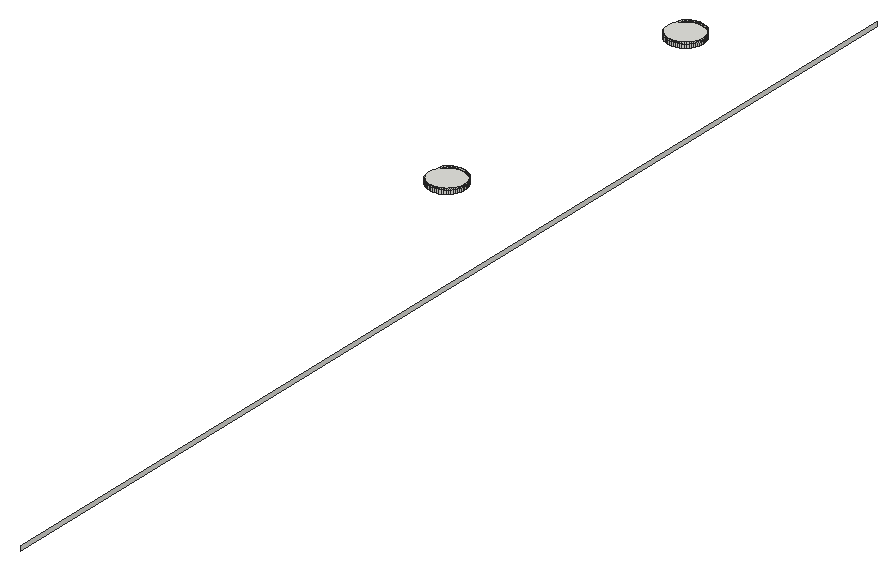
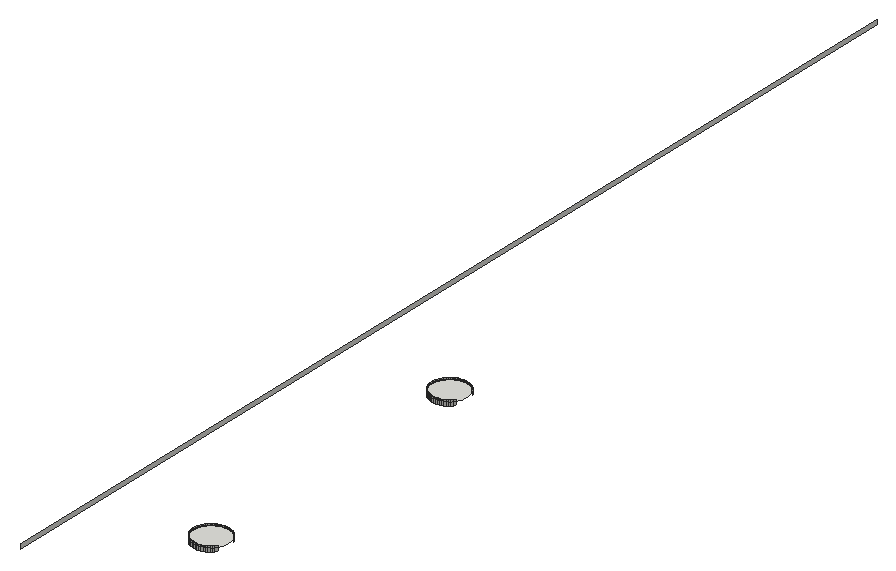
# SketchUp Ruby script. Lengths in inches.
U = 1.inch
M = Sketchup.active_model
def pt(a) = Geom::Point3d.new(a.map { |v| v * U })
def face(e, loops, mat)
  f = e.add_face(loops[0].map { |a| pt(a) })
  loops[1..].each { |l| e.add_face(l.map { |a| pt(a) }).erase! }
  f.material = f.back_material = mat if mat
  f
end
# faces: each face lists its corners as indices into pts; further lists are holes
def faces(e, pts, list, mat = nil) = list.each { |f| face(e, (f[0].is_a?(Array) ? f : [f]).map { |l| l.map { |i| pts[i] } }, mat) }
# xy, xz, yz: faces in a plane at the given z, y or x. An outline is a flat list of corners, or four numbers for a rectangle; further outlines are holes
def ring(l) = l.size == 4 ? [[l[0], l[1]], [l[2], l[1]], [l[2], l[3]], [l[0], l[3]]] : l.each_slice(2).to_a
def flat(e, list, mat, &to3) = list.each { |f| face(e, (f[0].is_a?(Array) ? f : [f]).map { |l| ring(l).map { |u, v| to3.(u, v) } }, mat) }
def xy(e, z, list, mat = nil) = flat(e, list, mat) { |x, y| [x, y, z] }
def xz(e, y, list, mat = nil) = flat(e, list, mat) { |x, z| [x, y, z] }
def yz(e, x, list, mat = nil) = flat(e, list, mat) { |y, z| [x, y, z] }
def lines(e, pts, list) = list.each { |a, b| e.add_line(pt(pts[a]), pt(pts[b])) }
# prism: a flat outline (further loops are holes) pulled along v
def prism(e, loops, v, mat = nil)
  f = face(e, loops, mat); d = Geom::Vector3d.new(v.map { |x| x * U })
  f.pushpull(f.normal.samedirection?(d) ? d.length : -d.length)
end
def box(e, o, s, mat = nil) = prism(e, [[o, [o[0] + s[0], o[1], o[2]], [o[0] + s[0], o[1] + s[1], o[2]], [o[0], o[1] + s[1], o[2]]]], [0, 0, s[2]], mat)
def at(x, y, z, deg = 0) = Geom::Transformation.translation(pt([x, y, z])) * Geom::Transformation.rotation(ORIGIN, Z_AXIS, deg.degrees)
def axes(o, x, y, z) = Geom::Transformation.new([*x, 0, *y, 0, *z, 0, *pt(o).to_a, 1])
def part(name) = M.definitions.add(name)
# library, detail: a bought-in or finely detailed component or shape, given as its bounding box
def library(name, o, s) = part(name).tap { |d| box(d.entities, o, s) }
def detail(e, o, s) = box(e.add_group.entities, o, s)
def put(e, d, t, mat = nil) = e.add_instance(d, t).tap { |i| i.material = mat if mat }
def group(e, t, mat = nil) = e.add_group.tap { |g| g.transformation = t; g.material = mat if mat }.entities
root = M.entities
xy(root,114.32,[[112.02,72.83,111.82,72.84,111.61,72.87,111.41,72.92,111.21,72.99,111.02,73.08,110.84,73.2,110.68,73.33,110.53,73.47,110.4,73.63,110.28,73.81,110.18,73.99,110.11,74.1875,110.05,74.39,110.01,74.59,110,74.8,110.01,75.01,110.04,75.22,110.09,75.42,110.16,75.62,110.26,75.81,110.37,75.98,110.5,76.15,110.64,76.3,110.8,76.43,110.98,76.55,111.16,76.65,111.36,76.72,111.56,76.78,111.77,76.8125,111.98,76.83,112.18,76.82,112.39,76.79,112.59,76.74,112.79,76.67,112.98,76.57,113.16,76.46,113.32,76.33,113.47,76.18,113.6,76.02,113.72,75.85,113.82,75.66,113.89,75.47,113.95,75.27,113.99,75.0625,114,74.85,113.99,74.64,113.96,74.4375,113.91,74.23,113.84,74.04,113.74,73.85,113.63,73.67,113.5,73.51,113.36,73.36,113.2,73.22,113.02,73.11,112.84,73.01,112.64,72.93,112.44,72.88,112.23,72.84],[112.02,106.24,111.82,106.25,111.61,106.28,111.41,106.33,111.21,106.41,111.02,106.5,110.84,106.61,110.68,106.74,110.53,106.89,110.4,107.05,110.28,107.22,110.18,107.41,110.11,107.6,110.05,107.8,110.01,108.01,110,108.22,110.01,108.43,110.04,108.63,110.09,108.84,110.16,109.03,110.26,109.22,110.37,109.4,110.5,109.5625,110.64,109.71,110.8,109.85,110.98,109.96,111.16,110.06,111.36,110.14,111.56,110.19,111.77,110.23,111.98,110.24,112.18,110.23,112.39,110.2,112.59,110.15,112.79,110.08,112.98,109.99,113.16,109.875,113.32,109.74,113.47,109.6,113.6,109.4375,113.72,109.26,113.82,109.08,113.89,108.88,113.95,108.68,113.99,108.48,114,108.27,113.99,108.06,113.96,107.85,113.91,107.65,113.84,107.45,113.74,107.26,113.63,107.09,113.5,106.92,113.36,106.77,113.2,106.64,113.02,106.52,112.84,106.43,112.64,106.35,112.44,106.29,112.23,106.26]])
yz(root,124,[[0,114,120,114.47]])
p = [[111.82,72.84,113.9],[111.61,72.87,113.9],[111.61,72.87,114.32],[111.82,72.84,114.32],[112.02,72.83,113.9],[112.02,72.83,114.32],
  [112.23,72.84,113.9],[112.23,72.84,114.32],[112.44,72.88,113.9],[112.44,72.88,114.32],[111.41,72.92,113.9],[111.21,72.99,113.9],
  [111.21,72.99,114.32],[111.41,72.92,114.32],[112.64,72.93,113.9],[112.64,72.93,114.32],[112.84,73.01,113.9],[112.84,73.01,114.32],
  [111.02,73.08,113.9],[111.02,73.08,114.32],[113.02,73.11,113.9],[113.02,73.11,114.32],[110.84,73.2,113.9],[110.84,73.2,114.32],
  [113.2,73.22,113.9],[113.2,73.22,114.32],[110.68,73.33,113.9],[110.68,73.33,114.32],[113.36,73.36,113.9],[113.36,73.36,114.32],
  [110.53,73.47,113.9],[110.53,73.47,114.32],[113.5,73.51,113.9],[113.5,73.51,114.32],[110.4,73.63,113.9],[110.4,73.63,114.32],
  [113.63,73.67,113.9],[113.63,73.67,114.32],[113.74,73.85,113.9],[113.74,73.85,114.32],[113.84,74.04,113.9],[113.84,74.04,114.32],
  [113.91,74.23,113.9],[113.91,74.23,114.32],[113.96,74.4375,113.9],[113.96,74.4375,114.32],[113.99,74.64,113.9],[113.99,74.64,114.32],
  [114,74.85,113.9],[114,74.85,114.32],[113.99,75.0625,113.9],[113.99,75.0625,114.32],[113.95,75.27,113.9],[113.95,75.27,114.32],
  [113.89,75.47,113.9],[113.89,75.47,114.32],[113.82,75.66,113.9],[113.82,75.66,114.32],[113.72,75.85,113.9],[113.72,75.85,114.32],
  [113.6,76.02,113.9],[113.6,76.02,114.32],[110.37,75.98,113.9],[110.5,76.15,113.9],[110.5,76.15,114.32],[110.37,75.98,114.32],
  [113.47,76.18,113.9],[113.47,76.18,114.32],[110.64,76.3,113.9],[110.64,76.3,114.32],[113.32,76.33,113.9],[113.32,76.33,114.32],
  [110.8,76.43,113.9],[110.8,76.43,114.32],[113.16,76.46,113.9],[113.16,76.46,114.32],[110.98,76.55,113.9],[110.98,76.55,114.32],
  [111.16,76.65,113.9],[111.16,76.65,114.32],[112.98,76.57,113.9],[112.98,76.57,114.32],[111.36,76.72,113.9],[111.36,76.72,114.32],
  [112.79,76.67,113.9],[112.79,76.67,114.32],[111.56,76.78,113.9],[111.56,76.78,114.32],[112.39,76.79,113.9],[112.59,76.74,113.9],
  [112.59,76.74,114.32],[112.39,76.79,114.32],[111.77,76.8125,113.9],[111.77,76.8125,114.32],[111.98,76.83,113.9],[111.98,76.83,114.32],
  [112.18,76.82,113.9],[112.18,76.82,114.32],[112.02,106.24,113.9],[111.82,106.25,113.9],[111.82,106.25,114.32],[112.02,106.24,114.32],
  [112.23,106.26,113.9],[112.23,106.26,114.32],[111.41,106.33,113.9],[111.21,106.41,113.9],[111.21,106.41,114.32],[111.41,106.33,114.32],
  [111.61,106.28,113.9],[111.61,106.28,114.32],[112.44,106.29,113.9],[112.44,106.29,114.32],[112.64,106.35,113.9],[112.64,106.35,114.32],
  [112.84,106.43,113.9],[112.84,106.43,114.32],[111.02,106.5,113.9],[111.02,106.5,114.32],[113.02,106.52,113.9],[113.02,106.52,114.32],
  [110.84,106.61,113.9],[110.84,106.61,114.32],[113.2,106.64,113.9],[113.2,106.64,114.32],[110.68,106.74,113.9],[110.68,106.74,114.32],
  [113.36,106.77,113.9],[113.36,106.77,114.32],[110.53,106.89,113.9],[110.53,106.89,114.32],[113.5,106.92,113.9],[113.5,106.92,114.32],
  [110.4,107.05,113.9],[110.4,107.05,114.32],[113.63,107.09,113.9],[113.63,107.09,114.32],[110.28,107.22,113.9],[110.28,107.22,114.32],
  [113.74,107.26,113.9],[113.74,107.26,114.32],[113.84,107.45,113.9],[113.84,107.45,114.32],[113.91,107.65,113.9],[113.91,107.65,114.32],
  [113.96,107.85,113.9],[113.96,107.85,114.32],[113.99,108.06,113.9],[113.99,108.06,114.32],[114,108.27,113.9],[114,108.27,114.32],
  [113.99,108.48,113.9],[113.99,108.48,114.32],[113.95,108.68,113.9],[113.95,108.68,114.32],[113.89,108.88,113.9],[113.89,108.88,114.32],
  [113.82,109.08,113.9],[113.82,109.08,114.32],[113.72,109.26,113.9],[113.72,109.26,114.32],[113.6,109.4375,113.9],[113.6,109.4375,114.32],
  [110.37,109.4,113.9],[110.5,109.5625,113.9],[110.5,109.5625,114.32],[110.37,109.4,114.32],[113.47,109.6,113.9],[113.47,109.6,114.32],
  [110.64,109.71,113.9],[110.64,109.71,114.32],[113.32,109.74,113.9],[113.32,109.74,114.32],[110.8,109.85,113.9],[110.8,109.85,114.32],
  [113.16,109.875,113.9],[113.16,109.875,114.32],[110.98,109.96,113.9],[110.98,109.96,114.32],[112.98,109.99,113.9],[112.98,109.99,114.32],
  [111.16,110.06,113.9],[111.16,110.06,114.32],[112.79,110.08,113.9],[112.79,110.08,114.32],[111.36,110.14,113.9],[111.36,110.14,114.32],
  [111.56,110.19,113.9],[111.56,110.19,114.32],[112.59,110.15,113.9],[112.59,110.15,114.32],[111.77,110.23,113.9],[111.77,110.23,114.32],
  [111.98,110.24,113.9],[111.98,110.24,114.32],[112.18,110.23,113.9],[112.18,110.23,114.32],[112.39,110.2,113.9],[112.39,110.2,114.32],
  [111.82,72.84,114.47],[111.61,72.87,114.47],[112.02,72.83,114.47],[112.23,72.84,114.47],[112.44,72.88,114.47],[111.41,72.92,114.47],
  [111.21,72.99,114.47],[112.64,72.93,114.47],[112.84,73.01,114.47],[111.02,73.08,114.47],[113.02,73.11,114.47],[110.84,73.2,114.47],
  [113.2,73.22,114.47],[110.68,73.33,114.47],[113.36,73.36,114.47],[110.53,73.47,114.47],[113.5,73.51,114.47],[110.4,73.63,114.47],
  [113.63,73.67,114.47],[110.28,73.81,114.32],[110.28,73.81,114.47],[113.74,73.85,114.47],[113.84,74.04,114.47],[113.91,74.23,114.47],
  [113.96,74.4375,114.47],[113.99,74.64,114.47],[114,74.85,114.47],[113.99,75.0625,114.47],[113.95,75.27,114.47],[113.89,75.47,114.47],
  [113.82,75.66,114.47],[113.72,75.85,114.47],[113.6,76.02,114.47],[110.37,75.98,114.47],[110.5,76.15,114.47],[113.47,76.18,114.47],
  [110.64,76.3,114.47],[113.32,76.33,114.47],[110.8,76.43,114.47],[113.16,76.46,114.47],[110.98,76.55,114.47],[111.16,76.65,114.47],
  [112.98,76.57,114.47],[111.36,76.72,114.47],[112.79,76.67,114.47],[111.56,76.78,114.47],[112.39,76.79,114.47],[112.59,76.74,114.47],
  [111.77,76.8125,114.47],[111.98,76.83,114.47],[112.18,76.82,114.47],[112.02,106.24,114.47],[111.82,106.25,114.47],[112.23,106.26,114.47],
  [111.41,106.33,114.47],[111.21,106.41,114.47],[111.61,106.28,114.47],[112.44,106.29,114.47],[112.64,106.35,114.47],[112.84,106.43,114.47],
  [111.02,106.5,114.47],[113.02,106.52,114.47],[110.84,106.61,114.47],[113.2,106.64,114.47],[110.68,106.74,114.47],[113.36,106.77,114.47],
  [110.53,106.89,114.47],[113.5,106.92,114.47],[110.4,107.05,114.47],[113.63,107.09,114.47],[110.28,107.22,114.47],[113.74,107.26,114.47],
  [113.84,107.45,114.47],[113.91,107.65,114.47],[113.96,107.85,114.47],[113.99,108.06,114.47],[114,108.27,114.47],[113.99,108.48,114.47],
  [113.95,108.68,114.47],[113.89,108.88,114.47],[113.82,109.08,114.47],[113.72,109.26,114.47],[113.6,109.4375,114.47],[110.37,109.4,114.47],
  [110.5,109.5625,114.47],[113.47,109.6,114.47],[110.64,109.71,114.47],[113.32,109.74,114.47],[110.8,109.85,114.47],[113.16,109.875,114.47],
  [110.98,109.96,114.47],[112.98,109.99,114.47],[111.16,110.06,114.47],[112.79,110.08,114.47],[111.36,110.14,114.47],[111.56,110.19,114.47],
  [112.59,110.15,114.47],[111.77,110.23,114.47],[111.98,110.24,114.47],[112.18,110.23,114.47],[112.39,110.2,114.47]]
faces(root,p,[[0,1,2,3],[4,0,3,5],[6,4,5,7],[8,6,7,9],[10,11,12,13],[1,10,13,2],[14,8,9,15],[16,14,15,17],
  [11,18,19,12],[20,16,17,21],[18,22,23,19],[24,20,21,25],[22,26,27,23],[28,24,25,29],[26,30,31,27],[32,28,29,33],
  [30,34,35,31],[36,32,33,37],[38,36,37,39],[40,38,39,41],[42,40,41,43],[44,42,43,45],[46,44,45,47],[48,46,47,49],
  [50,48,49,51],[52,50,51,53],[54,52,53,55],[56,54,55,57],[58,56,57,59],[60,58,59,61],[62,63,64,65],[66,60,61,67],
  [63,68,69,64],[70,66,67,71],[68,72,73,69],[74,70,71,75],[72,76,77,73],[76,78,79,77],[80,74,75,81],[78,82,83,79],
  [84,80,81,85],[82,86,87,83],[88,89,90,91],[89,84,85,90],[86,92,93,87],[92,94,95,93],[94,96,97,95],[96,88,91,97],
  [98,99,100,101],[102,98,101,103],[104,105,106,107],[108,104,107,109],[99,108,109,100],[110,102,103,111],[112,110,111,113],[114,112,113,115],
  [105,116,117,106],[118,114,115,119],[116,120,121,117],[122,118,119,123],[120,124,125,121],[126,122,123,127],[124,128,129,125],[130,126,127,131],
  [128,132,133,129],[134,130,131,135],[132,136,137,133],[138,134,135,139],[140,138,139,141],[142,140,141,143],[144,142,143,145],[146,144,145,147],
  [148,146,147,149],[150,148,149,151],[152,150,151,153],[154,152,153,155],[156,154,155,157],[158,156,157,159],[160,158,159,161],[162,163,164,165],
  [166,160,161,167],[163,168,169,164],[170,166,167,171],[168,172,173,169],[174,170,171,175],[172,176,177,173],[178,174,175,179],[176,180,181,177],
  [182,178,179,183],[180,184,185,181],[184,186,187,185],[188,182,183,189],[186,190,191,187],[190,192,193,191],[192,194,195,193],[194,196,197,195],
  [196,188,189,197],[198,3,2,199],[200,5,3,198],[201,7,5,200],[202,9,7,201],[203,13,12,204],[199,2,13,203],[205,15,9,202],
  [206,17,15,205],[204,12,19,207],[208,21,17,206],[207,19,23,209],[210,25,21,208],[209,23,27,211],[212,29,25,210],[211,27,31,213],
  [214,33,29,212],[213,31,35,215],[216,37,33,214],[215,35,217,218],[219,39,37,216],[220,41,39,219],[221,43,41,220],[222,45,43,221],
  [223,47,45,222],[224,49,47,223],[225,51,49,224],[226,53,51,225],[227,55,53,226],[228,57,55,227],[229,59,57,228],[230,61,59,229],
  [231,65,64,232],[233,67,61,230],[232,64,69,234],[235,71,67,233],[234,69,73,236],[237,75,71,235],[236,73,77,238],[238,77,79,239],
  [240,81,75,237],[239,79,83,241],[242,85,81,240],[241,83,87,243],[244,91,90,245],[245,90,85,242],[243,87,93,246],[246,93,95,247],
  [247,95,97,248],[248,97,91,244],[249,101,100,250],[251,103,101,249],[252,107,106,253],[254,109,107,252],[250,100,109,254],[255,111,103,251],
  [256,113,111,255],[257,115,113,256],[253,106,117,258],[259,119,115,257],[258,117,121,260],[261,123,119,259],[260,121,125,262],[263,127,123,261],
  [262,125,129,264],[265,131,127,263],[264,129,133,266],[267,135,131,265],[266,133,137,268],[269,139,135,267],[270,141,139,269],[271,143,141,270],
  [272,145,143,271],[273,147,145,272],[274,149,147,273],[275,151,149,274],[276,153,151,275],[277,155,153,276],[278,157,155,277],[279,159,157,278],
  [280,161,159,279],[281,165,164,282],[283,167,161,280],[282,164,169,284],[285,171,167,283],[284,169,173,286],[287,175,171,285],[286,173,177,288],
  [289,179,175,287],[288,177,181,290],[291,183,179,289],[290,181,185,292],[292,185,187,293],[294,189,183,291],[293,187,191,295],[295,191,193,296],
  [296,193,195,297],[297,195,197,298],[298,197,189,294]])
